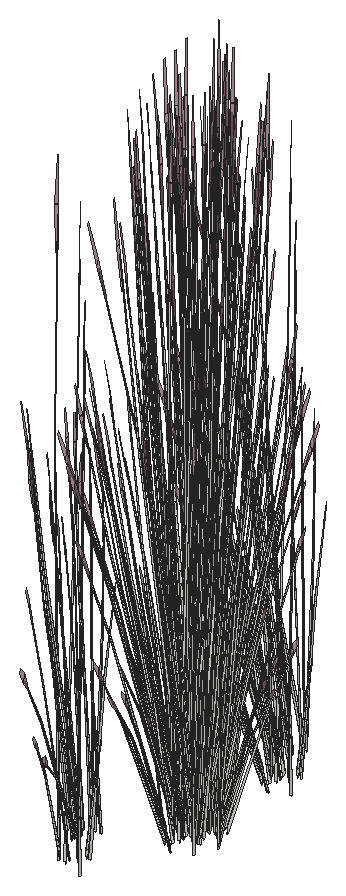
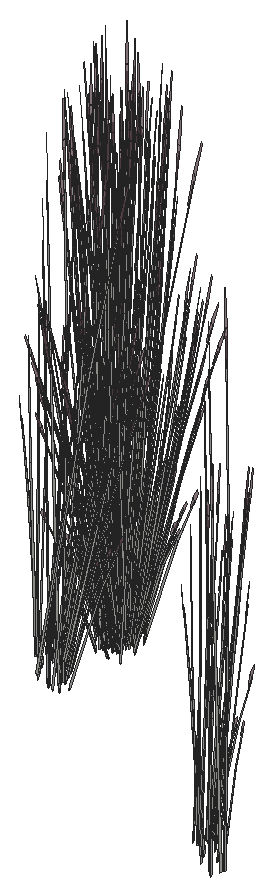
# SketchUp Ruby script. Lengths in inches.
U = 1.inch
M = Sketchup.active_model
def pt(a) = Geom::Point3d.new(a.map { |v| v * U })
def face(e, loops, mat)
  f = e.add_face(loops[0].map { |a| pt(a) })
  loops[1..].each { |l| e.add_face(l.map { |a| pt(a) }).erase! }
  f.material = f.back_material = mat if mat
  f
end
# faces: each face lists its corners as indices into pts; further lists are holes
def faces(e, pts, list, mat = nil) = list.each { |f| face(e, (f[0].is_a?(Array) ? f : [f]).map { |l| l.map { |i| pts[i] } }, mat) }
# xy, xz, yz: faces in a plane at the given z, y or x. An outline is a flat list of corners, or four numbers for a rectangle; further outlines are holes
def ring(l) = l.size == 4 ? [[l[0], l[1]], [l[2], l[1]], [l[2], l[3]], [l[0], l[3]]] : l.each_slice(2).to_a
def flat(e, list, mat, &to3) = list.each { |f| face(e, (f[0].is_a?(Array) ? f : [f]).map { |l| ring(l).map { |u, v| to3.(u, v) } }, mat) }
def xy(e, z, list, mat = nil) = flat(e, list, mat) { |x, y| [x, y, z] }
def xz(e, y, list, mat = nil) = flat(e, list, mat) { |x, z| [x, y, z] }
def yz(e, x, list, mat = nil) = flat(e, list, mat) { |y, z| [x, y, z] }
def lines(e, pts, list) = list.each { |a, b| e.add_line(pt(pts[a]), pt(pts[b])) }
# prism: a flat outline (further loops are holes) pulled along v
def prism(e, loops, v, mat = nil)
  f = face(e, loops, mat); d = Geom::Vector3d.new(v.map { |x| x * U })
  f.pushpull(f.normal.samedirection?(d) ? d.length : -d.length)
end
def box(e, o, s, mat = nil) = prism(e, [[o, [o[0] + s[0], o[1], o[2]], [o[0] + s[0], o[1] + s[1], o[2]], [o[0], o[1] + s[1], o[2]]]], [0, 0, s[2]], mat)
def at(x, y, z, deg = 0) = Geom::Transformation.translation(pt([x, y, z])) * Geom::Transformation.rotation(ORIGIN, Z_AXIS, deg.degrees)
def axes(o, x, y, z) = Geom::Transformation.new([*x, 0, *y, 0, *z, 0, *pt(o).to_a, 1])
def part(name) = M.definitions.add(name)
# library, detail: a bought-in or finely detailed component or shape, given as its bounding box
def library(name, o, s) = part(name).tap { |d| box(d.entities, o, s) }
def detail(e, o, s) = box(e.add_group.entities, o, s)
def put(e, d, t, mat = nil) = e.add_instance(d, t).tap { |i| i.material = mat if mat }
def group(e, t, mat = nil) = e.add_group.tap { |g| g.transformation = t; g.material = mat if mat }.entities
root = M.entities
M.materials.add("LightPink_Translucent").color = [144, 107, 117]
M.materials["LightPink_Translucent"].alpha = 0.75
c1 = part("blade")
p = [[2.15,0.21,22],[0,0.17,0],[0.09,0.45,0],[2.18,0.31,22],[2.29,0.31,22],[0.38,0.45,0],
  [2.48,0.24,33],[2.49,0.24,33],[2.48,0.22,33]]
faces(c1.entities,p,[[0,1,2,3],[4,5,2,3],[6,3,4,7],[8,0,3,6]])
c2 = part("seeds")
p = [[0.3,-0.1,1.38],[-0.01,-0.03,1.59],[-0.01,-0.03,0.03],[0.14,-0.07,-0.07],[0.29,-0.03,3],[0.15,0.01,3.11]]
faces(c2.entities,p,[[0,1,2,3],[1,0,4,5]],"LightPink_Translucent")
c3 = part("blade with seeds")
put(c3.entities,c1,at(0,0,0))
put(c3.entities,c2,axes([2.4,0.25,30.99],[1.5799,-0.05474,1.17369],[-0.12525,1.92788,0.29478],[-0.07173,-0.02425,1.56792]))
put(root,c3,axes([401.27,9.57,3.875],[0.08068,0.14973,1.71376],[-0.3728,0.12606,0.13857],[-0.08426,-0.23506,0.73262]))
put(root,c3,axes([402.72,9.36,2.59],[-0.10032,0.0944,1.43002],[-0.30046,-0.16522,-0.30754],[0.05569,-0.20547,0.61141]))
put(root,c3,axes([402.27,9.68,4.98],[-0.16845,-0.3792,-0.71045],[0.34676,-0.21133,0.08574],[-0.03939,-0.18322,1.00501]))
put(root,c3,axes([401.17,9.18,2.59],[-0.02137,0.15256,1.43002],[-0.31245,0.12771,-0.30754],[-0.07303,-0.19719,0.61141]))
put(root,c3,axes([401.98,8.84,1.49],[-0.0592,0.0168,1.76342],[-0.32738,-0.18913,-0.26939],[0.00549,-0.15776,0.30037]))
put(root,c3,axes([402.97,10.06,4.98],[0.00918,-0.43138,-0.71045],[0.38672,0.02897,0.08574],[0.04081,-0.18275,1.00501]))
put(root,c3,axes([402.3,9.36,4.53],[0.1064,-0.35863,-0.35414],[0.31043,0.1046,0.4572],[-0.02846,-0.14439,0.87481]))
put(root,c3,axes([402.53,9.84,3.875],[-0.06572,0.16029,1.71376],[-0.27569,-0.33172,0.13857],[0.12437,-0.20675,0.73262]))
put(root,c3,axes([402.14,9.61,4.68],[-0.34695,-0.11691,-0.51099],[0.11892,-0.40083,-0.3958],[-0.03181,-0.16138,0.97773]))
put(root,c3,axes([402.35,8.6,2.77],[0.04528,0.27194,1.1486],[-0.25117,-0.15062,0.84392],[0.02703,-0.13924,0.25299]))
put(root,c3,axes([402.89,9.91,4.68],[-0.25266,-0.31335,-0.51099],[0.2669,-0.27442,-0.3958],[0.03844,-0.15921,0.97773]))
put(root,c3,axes([403.13,9.8,4.53],[0.23881,-0.24554,-0.35414],[0.22606,0.28036,0.4572],[0.0344,-0.14245,0.87481]))
put(root,c3,axes([401.0625,8.93,2.77],[0.18411,0.16231,1.1486],[-0.26813,0.09757,0.84392],[-0.05737,-0.12474,0.25299]))
put(root,c3,axes([401.51,9.79,4.98],[-0.30095,-0.22541,-0.71045],[0.21388,-0.395,0.08574],[-0.10904,-0.13459,1.00501]))
put(root,c3,axes([401.4,9.49,4.53],[-0.05451,-0.37564,-0.35414],[0.31161,-0.09919,0.4572],[-0.0837,-0.10765,0.87481]))
put(root,c3,axes([400.92,9.42,1.49],[-0.03419,0.06144,1.76342],[-0.3455,0.13246,-0.26939],[-0.08346,-0.12049,0.30037]))
put(root,c3,axes([401.49,11.11,2.1],[-0.14494,-0.47823,-0.69835],[0.41752,-0.17223,-0.18329],[-0.01602,-0.16194,1.54149]))
put(root,c3,axes([400.73,10.04,3.875],[0.1311,0.08035,1.71376],[-0.27131,0.33708,0.13857],[-0.16909,-0.15206,0.73262]))
put(root,c3,axes([403.43,9.65,1.49],[-0.05283,-0.03674,1.76342],[-0.13569,-0.41045,-0.26939],[0.09154,-0.11138,0.30037]))
put(root,c3,axes([401.37,9.8,4.68],[-0.34827,0.11086,-0.51099],[-0.06092,-0.41983,-0.3958],[-0.09354,-0.12031,0.97773]))
put(root,c3,axes([403.42,10.81,4.98],[0.18436,-0.36797,-0.71045],[0.32306,0.26151,0.08574],[0.11008,-0.13332,1.00501]))
put(root,c3,axes([401.43,9.73,2.375],[-0.22066,-0.46731,0],[0.36918,-0.26061,-0.51607],[0.08408,-0.05936,1.63711]))
put(root,c3,axes([403.41,10.63,4.68],[-0.09067,-0.42583,-0.51099],[0.34336,-0.07449,-0.3958],[0.0984,-0.11438,0.97773]))
put(root,c3,axes([401.92,9.17,2.13],[-0.2439,0.26754,-0.03893],[-0.22348,-0.29302,-0.17649],[-0.01573,-0.08303,0.58215]))
put(root,c3,axes([402.23,12.34,3.33],[0.305,0.18805,1.51261],[-0.29879,0.40513,0.59816],[-0.13384,-0.24012,1.26806]))
put(root,c3,axes([400.63,11.04,2.02],[0,-0.46636,-0.49651],[0.39487,0,0],[0,-0.10622,1.57504]))
put(root,c3,axes([401.73,9.66,2.02],[0.33032,-0.23318,-0.49651],[0.19744,0.41812,0],[0.07523,-0.05311,1.57504]))
put(root,c3,axes([403.69,10.47,2.59],[-0.12609,-0.01381,1.43002],[-0.12917,-0.37055,-0.30754],[0.1549,-0.10482,0.61141]))
put(root,c3,axes([402.12,10.62,2.06],[0.23773,-0.35053,-0.62353],[0.29532,0.31785,-0.16365],[0.09526,-0.08744,1.37633]))
put(root,c3,axes([403.84,9.79,2.77],[-0.11756,0.2374,1.1486],[-0.10105,-0.31895,0.84392],[0.09709,-0.07992,0.25299]))
put(root,c3,axes([403.67,10.68,4.53],[0.30722,-0.06665,-0.35414],[0.08112,0.381,0.4572],[0.08804,-0.10234,0.87481]))
put(root,c3,axes([401.71,11.23,2.21],[0.17124,-0.42022,-0.44739],[0.35581,0.20224,0.21531],[0,-0.09687,1.43643]))
put(root,c3,axes([400.68,10.15,4.53],[-0.20082,-0.29199,-0.35414],[0.2293,-0.2764,0.4572],[-0.1165,-0.04206,0.87481]))
put(root,c3,axes([401.86,11.02,2.67],[-0.04113,-0.53214,-0.29095],[0.42835,-0.03218,-0.50002],[0.07543,-0.07088,1.59708]))
put(root,c3,axes([400.8,11.05,2.03],[0.24637,-0.29097,-0.30978],[0.24637,0.29097,0.30978],[0,-0.09372,1.38974]))
put(root,c3,axes([400.7,9.66,2.13],[-0.10181,0.3808,-0.03893],[-0.31336,-0.11714,-0.17649],[-0.04758,-0.06228,0.58215]))
put(root,c3,axes([401.67,11.58,2.67],[-0.39748,-0.22252,-0.29095],[0.19139,-0.46966,-0.50002],[-0.01249,-0.11531,1.59708]))
put(root,c3,axes([400.53,11.4,2.375],[-0.44133,0,0],[0,-0.52122,-0.51607],[0,-0.11871,1.63711]))
put(root,c3,axes([400.61,10.46,2.59],[0.06891,0.12984,1.43002],[-0.15879,0.35293,-0.30754],[-0.16304,-0.08436,0.61141]))
put(root,c3,axes([401.81,9.85,2.03],[0.32928,0.11539,-0.30978],[-0.08291,0.40636,0.30978],[0.06638,-0.04686,1.38974]))
put(root,c3,axes([400.89,10.35,4.98],[-0.35281,-0.01123,-0.71045],[0.0237,-0.47284,0.08574],[-0.14947,-0.0499,1.00501]))
put(root,c3,axes([400.875,11.26,2.33],[-0.32829,0.39208,0.30756],[-0.32849,-0.38796,-0.36492],[-0.01146,-0.11134,1.64885]))
put(root,c3,axes([401.92,11.44,2.43],[0.39767,0.22603,0.24065],[-0.19139,0.46966,0.50002],[0,-0.10827,1.60543]))
put(root,c3,axes([401.77,12.08,2.4375],[0.09355,-0.55261,-0.23429],[0.44354,0.09633,0.51271],[-0.0775,-0.07631,1.5644]))
put(root,c3,axes([400.78,10.45,4.68],[-0.25628,0.30892,-0.51099],[-0.22444,-0.32634,-0.3958],[-0.13021,-0.047,0.97773]))
put(root,c3,axes([400.2,10.85,2.77],[0.22533,-0.03337,1.1486],[-0.14293,0.29403,0.84392],[-0.11135,-0.04411,0.25299]))
put(root,c3,axes([401.79,11.125,2.72],[-0.38326,0.02879,0.44739],[-0.03466,-0.47788,-0.21531],[0.06861,-0.04843,1.43643]))
put(root,c3,axes([400.8,11.48,2.48],[0,0.46636,0.49651],[-0.39487,0,0],[0,-0.10622,1.57504]))
put(root,c3,axes([403.57,11.58,4.68],[0.09562,-0.42421,-0.51099],[0.32782,0.1454,-0.3958],[0.13199,-0.0389,0.97773]))
put(root,c3,axes([403.06,9.85,2.375],[0.22066,-0.46731,0],[0.36918,0.26061,-0.51607],[0.08408,0.05936,1.63711]))
put(root,c3,axes([400.46,10.78,3.875],[0.14639,-0.01056,1.71376],[-0.09712,0.45778,0.13857],[-0.20862,-0.02831,0.73262]))
put(root,c3,axes([401.73,11.85,2.21],[-0.21202,-0.39143,-0.44739],[0.32115,-0.27564,0.21531],[-0.06861,-0.04843,1.43643]))
put(root,c3,axes([401.78,11.3,2.36],[0.15345,0.52148,0.45755],[-0.43845,0.18134,0.17955],[0.00536,-0.09582,1.58856]))
put(root,c3,axes([403.92,11.7,1.98],[-0.22732,0.05597,1.41583],[-0.03618,-0.44548,0.08104],[0.15921,-0.06743,0.80566]))
put(root,c3,axes([404.34,11.3,2.26],[-0.21881,-0.29821,-0.06488],[0.23965,-0.27324,-0.29416],[0.0679,-0.01924,0.97024]))
put(root,c3,axes([401.7,11.71,2.72],[-0.17124,0.42022,0.44739],[-0.35581,-0.20224,-0.21531],[0,-0.09687,1.43643]))
put(root,c3,axes([402.33,11.34,2.21],[0,-0.53961,0],[0.44133,0,0],[0,0,1.79456]))
put(root,c3,axes([402.87,10.1,2.48],[-0.33032,-0.23318,0.49651],[0.19744,-0.41812,0],[0.07523,0.05311,1.57504]))
put(root,c3,axes([403.51,11.73,4.98],[0.31014,-0.20596,-0.71045],[0.17284,0.42397,0.08574],[0.14985,-0.04816,1.00501]))
put(root,c3,axes([401.54,12,2.06],[-0.36714,-0.07646,-0.62353],[0.07747,-0.47163,-0.16365],[-0.10956,-0.05715,1.37633]))
put(root,c3,axes([402.12,11,2.36],[-0.29264,0.42323,0.45755],[-0.34767,-0.3736,0.17955],[0.07055,-0.04224,1.58856]))
put(root,c3,axes([402.44,11.76,2.3],[-0.32829,-0.4014,-0.06131],[0.32849,-0.40164,0],[-0.01146,-0.01402,1.75571]))
put(root,c3,axes([401.61,10.31,2.47],[-0.10196,0.46348,0.17642],[-0.3731,-0.13116,0.35086],[0.06445,-0.00226,1.60407]))
put(root,c3,axes([401.46,10.68,1.59],[-0.3474,0.18671,1.28929],[-0.11057,-0.53572,0.50096],[0.21332,0.00891,1.46642]))
put(root,c3,axes([402.39,10.82,2.62],[0.06809,-0.4162,0.1448],[0.33266,0.07225,-0.41347],[0.06054,0.04274,1.26744]))
put(root,c3,axes([401.82,11.81,2.36],[0.44609,0.09826,0.45755],[-0.09078,0.55493,0.17955],[-0.06519,-0.05359,1.58856]))
put(root,c3,axes([404.17,11.41,1.49],[-0.01845,-0.0708,1.76342],[0.12793,-0.41416,-0.26939],[0.12905,-0.00596,0.30037]))
put(root,c3,axes([400.36,11.34,1.49],[0.00895,0.0735,1.76342],[-0.18044,0.38382,-0.26939],[-0.12817,-0.01935,0.30037]))
put(root,c3,axes([402.25,10.93,2.72],[-0.21202,-0.39143,0.44739],[0.32115,-0.27564,-0.21531],[0.06861,0.04843,1.43643]))
put(root,c3,axes([401.15,12.72,2.03],[-0.08291,-0.40636,-0.30978],[0.32928,-0.11539,0.30978],[-0.06638,-0.04686,1.38974]))
put(root,c3,axes([401.58,12.7,2.47],[0.37926,-0.12378,0.17642],[0.09365,0.46065,0.35086],[-0.03382,-0.06712,1.60407]))
put(root,c3,axes([402.36,10.96,2.67],[0.35635,-0.30962,-0.29095],[0.23697,0.43749,-0.50002],[0.08792,0.04443,1.59708]))
put(root,c3,axes([403.78,11.77,4.53],[0.29332,0.1301,-0.35414],[-0.08555,0.37955,0.4572],[0.11809,-0.0348,0.87481]))
put(root,c3,axes([401.0625,12.89,2.02],[-0.33032,-0.23318,-0.49651],[0.19744,-0.41812,0],[-0.07523,-0.05311,1.57504]))
put(root,c3,axes([403.26,10.13,2.02],[0.33032,0.23318,-0.49651],[-0.19744,0.41812,0],[0.07523,0.05311,1.57504]))
put(root,c3,axes([400.33,11.17,4.53],[-0.29332,-0.1301,-0.35414],[0.08555,-0.37955,0.4572],[-0.11809,0.0348,0.87481]))
put(root,c3,axes([402.63,11.46,2.21],[0.39487,0,0],[0,0.48281,0],[0,0,1.78407]))
put(root,c3,axes([401.96,12.07,2.67],[-0.35635,0.30962,-0.29095],[-0.23697,-0.43749,-0.50002],[-0.08792,-0.04443,1.59708]))
put(root,c3,axes([402.74,10.33,2.47],[-0.37926,0.12378,0.17642],[-0.09365,-0.46065,0.35086],[0.03382,0.06712,1.60407]))
put(root,c3,axes([402.98,11.3,3.875],[-0.14639,0.01056,1.71376],[0.09712,-0.45778,0.13857],[0.20862,0.02831,0.73262]))
put(root,c3,axes([403.17,10.31,2.03],[0.08291,0.40636,-0.30978],[-0.32928,0.11539,0.30978],[0.06638,0.04686,1.38974]))
put(root,c3,axes([402.5,11.22,2.38],[-0.44609,-0.09826,0.49198],[0.09078,-0.55493,0.19306],[0.06519,0.05359,1.70813]))
put(root,c3,axes([402.15,12.59,2.2],[-0.11516,-0.40207,0],[0.32884,-0.1408,0],[0,0,1.54371]))
put(root,c3,axes([401.93,12.21,2.62],[-0.06809,0.4162,0.1448],[-0.33266,-0.07225,-0.41347],[-0.06054,-0.04274,1.26744]))
put(root,c3,axes([402.58,12.53,2.18],[0.37054,-0.15823,-0.19198],[0.1302,0.45581,0.00008],[0.0409,-0.01749,1.73897]))
put(root,c3,axes([402.71,12.72,2.47],[0.10196,-0.46348,0.17642],[0.3731,0.13116,0.35086],[-0.06445,0.00226,1.60407]))
put(root,c3,axes([402.62,11.67,2.21],[0.24637,0.30123,0],[-0.24637,0.30123,0],[0,0,1.69266]))
put(root,c3,axes([401.22,11.1,3.34],[0.10032,-0.06746,1.77064],[0.0346,0.47103,0.13857],[-0.2173,0.0625,0.63284]))
put(root,c3,axes([403.29,11.54,2.47],[-0.2773,-0.3397,0.17642],[0.27945,-0.32949,0.35086],[-0.03063,0.06937,1.60407]))
put(root,c3,axes([402.78,11.03,2.06],[0.36714,0.07646,-0.62353],[-0.07747,0.47163,-0.16365],[0.10956,0.05715,1.37633]))
put(root,c3,axes([404.4,11.85,2.77],[-0.21807,0.07699,1.1486],[0.10265,-0.31819,0.84392],[0.11568,0.02177,0.25299]))
put(root,c3,axes([402.07,12.77,2.2],[-0.35581,-0.20937,0],[0.17124,-0.43505,0],[0,0,1.62707]))
put(root,c3,axes([402.36,12.21,2.46],[-0.34464,-0.37536,-0.25192],[0.29,-0.42149,0.5513],[-0.0928,0.04391,1.68216]))
put(root,c3,axes([401.45,12.93,2.48],[0.33032,0.23318,0.49651],[-0.19744,0.41812,0],[-0.07523,-0.05311,1.57504]))
put(root,c3,axes([402.62,11.32,2.72],[0.17124,-0.42022,0.44739],[0.35581,0.20224,-0.21531],[0,0.09687,1.43643]))
put(root,c3,axes([402.55,11.56,2.29],[0,0.53934,-0.05637],[-0.44133,0,0],[0,0.01695,1.79368]))
put(root,c3,axes([400.53,11.36,4.68],[-0.09562,0.42421,-0.51099],[-0.32782,-0.1454,-0.3958],[-0.13199,0.0389,0.97773]))
put(root,c3,axes([402.58,11.18,2.21],[0.21202,0.39143,-0.44739],[-0.32115,0.27564,0.21531],[0.06861,0.04843,1.43643]))
put(root,c3,axes([404.02,12.83,3.93],[-0.06755,-0.39203,-0.03492],[0.31928,-0.09013,-0.15832],[0.06667,0.02485,0.52218]))
put(root,c3,axes([401.26,13.18,2.375],[-0.22066,0.46731,0],[-0.36918,-0.26061,-0.51607],[-0.08408,-0.05936,1.63711]))
put(root,c3,axes([403.52,11.55,2.48],[0,-0.46636,0.49651],[0.39487,0,0],[0,0.10622,1.57504]))
put(root,c3,axes([402.53,11.9,2.72],[0.38326,-0.02879,0.44739],[0.03466,0.47788,-0.21531],[-0.06861,0.04843,1.43643]))
put(root,c3,axes([402.77,11.41,2.62],[0.32884,-0.136,0.1448],[0.11516,0.38837,-0.41347],[0,0.08547,1.26744]))
put(root,c3,axes([402.1875,12.13,2.21],[-0.38326,0.02879,-0.44739],[-0.03466,-0.47788,0.21531],[-0.06861,0.04843,1.43643]))
put(root,c3,axes([403.99,12.36,2.59],[-0.085,-0.1147,1.43002],[0.1106,-0.37943,-0.30754],[0.17198,0.0514,0.61141]))
put(root,c3,axes([402.47,12.78,2.2],[0.35581,0.20937,0],[-0.17124,0.43505,0],[0,0,1.74954]))
put(root,c3,axes([402.61,13.24,2.19],[-0.21791,-0.46895,-0.05142],[0.36918,-0.26061,0.51607],[-0.09097,0.04465,1.6363]))
put(root,c3,axes([402.53,12.11,2.62],[0.26075,0.2802,0.1448],[-0.2175,0.31612,-0.41347],[-0.06054,0.04274,1.26744]))
put(root,c3,axes([400.52,11.58,3.875],[0.12246,-0.09864,1.71376],[0.1031,0.45582,0.13857],[-0.19225,0.10302,0.73262]))
put(root,c3,axes([403.21,12.59,4.98],[0.35281,0.01123,-0.71045],[-0.0237,0.47284,0.08574],[0.14947,0.0499,1.00501]))
put(root,c3,axes([402.8125,12.97,2.48],[0.33032,-0.23318,0.49651],[0.19744,0.41812,0],[-0.07523,0.05311,1.57504]))
put(root,c3,axes([402.34,12.6,2.29],[0.15345,0.53576,-0.06012],[-0.43845,0.18773,0],[0.00536,0.01871,1.72173]))
put(root,c3,axes([402.51,13.18,2.03],[-0.32928,-0.11539,-0.30978],[0.08291,-0.40636,0.30978],[-0.06638,0.04686,1.38974]))
put(root,c3,axes([400.14,12.36,2.59],[0.12266,0.03828,1.43002],[0.07906,0.39104,-0.30754],[-0.16661,0.0732,0.61141]))
put(root,c3,axes([403.78,11.63,2.375],[0.44133,0,0],[0,0.52122,-0.51607],[0,0.11871,1.63711]))
put(root,c3,axes([403.61,11.9,2.2],[-0.44111,-0.00373,-0.04976],[0,-0.52122,0.49943],[-0.01386,0.11865,1.58352]))
put(root,c3,axes([402.65,11.45,2.67],[0.39748,0.22252,-0.29095],[-0.19139,0.46966,-0.50002],[0.01249,0.11531,1.59708]))
put(root,c3,axes([399.88,13.18,2.77],[0.14709,-0.21136,1.1486],[0.05804,0.3346,0.84392],[-0.1063,0.05991,0.25299]))
put(root,c3,axes([403.42,12.79,4.53],[0.20082,0.29199,-0.35414],[-0.2293,0.2764,0.4572],[0.1165,0.04206,0.87481]))
put(root,c3,axes([403.52,11.98,2.03],[-0.24637,0.29097,-0.30978],[-0.24637,-0.29097,0.30978],[0,0.09372,1.38974]))
put(root,c3,axes([402.46,12,2.67],[0.04113,0.53214,-0.29095],[-0.42835,0.03218,-0.50002],[-0.07543,0.07088,1.59708]))
put(root,c3,axes([402.61,11.8,2.21],[-0.17124,0.42022,-0.44739],[-0.35581,-0.20224,0.21531],[0,0.09687,1.43643]))
put(root,c3,axes([400.43,12.26,4.53],[-0.30722,0.06665,-0.35414],[-0.08112,-0.381,0.4572],[-0.08804,0.10234,0.87481]))
put(root,c3,axes([402.2,12.41,2.06],[-0.23773,0.35053,-0.62353],[-0.29532,-0.31785,-0.16365],[-0.09526,0.08744,1.37633]))
put(root,c3,axes([402.62,13,2.33],[0.44186,0.15158,0.30756],[-0.11054,0.54181,-0.36492],[-0.07313,0.06781,1.64885]))
put(root,c3,axes([402.59,13.37,2.02],[-0.33032,0.23318,-0.49651],[-0.19744,-0.41812,0],[-0.07523,0.05311,1.57504]))
put(root,c3,axes([403.6875,11.99,2.02],[0,0.46636,-0.49651],[-0.39487,0,0],[0,0.10622,1.57504]))
put(root,c3,axes([402.7,12.04,3.875],[-0.1311,-0.08035,1.71376],[0.27131,-0.33708,0.13857],[0.16909,0.15206,0.73262]))
put(root,c3,axes([403.18,12.95,2.77],[-0.19872,-0.13409,1.1486],[0.2566,-0.13625,0.84392],[0.06921,0.11541,0.25299]))
put(root,c3,axes([400.97,11.89,3.875],[0.08815,-0.14329,1.71376],[0.22258,0.38678,0.13857],[-0.15267,0.17614,0.73262]))
put(root,c3,axes([400.6875,12.31,4.68],[0.09067,0.42583,-0.51099],[-0.34336,0.07449,-0.3958],[-0.0984,0.11438,0.97773]))
put(root,c3,axes([402.89,13.29,2.375],[0.22066,0.46731,0],[-0.36918,0.26061,-0.51607],[-0.08408,0.05936,1.63711]))
put(root,c3,axes([403.24,13.45,1.49],[0.02571,-0.06733,1.76342],[0.32373,-0.19829,-0.26939],[0.09815,0.10263,0.30037]))
put(root,c3,axes([402.7,11.44,2.84],[-0.00964,-0.43909,1.41272],[0.43635,0.11382,0.59816],[-0.1032,0.24027,1.3335]))
put(root,c3,axes([402.8125,11.92,2.09],[0.12941,0.42699,-0.69212],[-0.37279,0.15378,-0.18165],[0.0143,0.14459,1.52773]))
put(root,c3,axes([400.27,13.39,1.49],[0.04734,0.04659,1.76342],[0.08027,0.4317,-0.26939],[-0.10492,0.09206,0.30037]))
put(root,c3,axes([402.74,13.14,4.68],[0.34827,-0.11086,-0.51099],[0.06092,0.41983,-0.3958],[0.09354,0.12031,0.97773]))
put(root,c3,axes([403.22,13.5625,2.67],[-0.22633,-0.01463,1.0506],[0.14947,-0.31064,0.58006],[0.08941,0.11036,0.8241]))
put(root,c3,axes([400.9,12.24,3.875],[0.06572,-0.16029,1.71376],[0.27569,0.33172,0.13857],[-0.12437,0.20675,0.73262]))
put(root,c3,axes([402.48,12.81,2.59],[0.00623,-0.15459,1.43002],[0.29764,-0.17268,-0.30754],[0.09188,0.18503,0.61141]))
put(root,c3,axes([400.98,13.14,4.53],[-0.23881,0.24554,-0.35414],[-0.22606,-0.28036,0.4572],[-0.0344,0.14245,0.87481]))
put(root,c3,axes([401.13,14.1,2.77],[-0.00913,-0.2773,1.1486],[0.22824,0.19778,0.84392],[-0.04489,0.13217,0.25299]))
put(root,c3,axes([401.73,13.4375,1.49],[0.05712,-0.02538,1.76342],[0.34359,0.13968,-0.26939],[0.01005,0.15742,0.30037]))
put(root,c3,axes([401.21,13.03,5],[0.25266,0.31335,-0.5672],[-0.2669,0.27442,-0.43934],[-0.03844,0.15921,1.08528]))
put(root,c3,axes([400.9375,13.5,2.82],[0.32063,-0.08258,0.06507],[0.07371,0.33271,-0.86304],[-0.02033,0.16842,0.7736]))
put(root,c3,axes([401.27,20.52,3.875],[0.08068,0.14973,1.71376],[-0.3728,0.12606,0.13857],[-0.08426,-0.23506,0.73262]))
put(root,c3,axes([401.96,13.33,4.68],[0.34695,0.11691,-0.51099],[-0.11892,0.40083,-0.3958],[0.03181,0.16138,0.97773]))
put(root,c3,axes([402.16,12.5,3.875],[-0.08068,-0.14973,1.71376],[0.3728,-0.12606,0.13857],[0.08426,0.23506,0.73262]))
put(root,c3,axes([383.7,20.3,-10.62],[-0.10032,0.0944,1.43002],[-0.30046,-0.16522,-0.30754],[0.05569,-0.20547,0.61141]))
put(root,c3,axes([402.72,20.3,2.59],[-0.10032,0.0944,1.43002],[-0.30046,-0.16522,-0.30754],[0.05569,-0.20547,0.61141]))
put(root,c3,axes([401.8,13.58,4.53],[-0.1064,0.35863,-0.35414],[-0.31043,-0.1046,0.4572],[0.02846,0.14439,0.87481]))
put(root,c3,axes([402.27,20.63,4.98],[-0.16845,-0.3792,-0.71045],[0.34676,-0.21133,0.08574],[-0.03939,-0.18322,1.00501]))
put(root,c3,axes([401.17,20.12,2.59],[-0.02137,0.15256,1.43002],[-0.31245,0.12771,-0.30754],[-0.07303,-0.19719,0.61141]))
put(root,c3,axes([401.13,12.89,5.34],[-0.00918,0.43138,-0.7886],[-0.38672,-0.02897,0.09517],[-0.04081,0.18275,1.11556]))
put(root,c3,axes([401.98,19.79,1.49],[-0.0592,0.0168,1.76342],[-0.32738,-0.18913,-0.26939],[0.00549,-0.15776,0.30037]))
put(root,c3,axes([401.5,12.58,3.875],[-0.00864,-0.17899,1.71376],[0.37441,0.11874,0.13857],[-0.02316,0.25508,0.73262]))
put(root,c3,axes([383.9375,21,-8.23],[0.00918,-0.43138,-0.71045],[0.38672,0.02897,0.08574],[0.04081,-0.18275,1.00501]))
put(root,c3,axes([402.97,21,4.98],[0.00918,-0.43138,-0.71045],[0.38672,0.02897,0.08574],[0.04081,-0.18275,1.00501]))
put(root,c3,axes([401.84,13.26,4.98],[0.16845,0.3792,-0.71045],[-0.34676,0.21133,0.08574],[0.03939,0.18322,1.00501]))
put(root,c3,axes([384.48,20.33,-8.5],[-0.00341,-0.09282,1.74944],[-0.28775,-0.26825,-0.27667],[0.04449,-0.16261,0.14031]))
put(root,c3,axes([402.3,20.31,4.53],[0.1064,-0.35863,-0.35414],[0.31043,0.1046,0.4572],[-0.02846,-0.14439,0.87481]))
put(root,c3,axes([383.5,20.78,-9.33],[-0.06572,0.16029,1.71376],[-0.27569,-0.33172,0.13857],[0.12437,-0.20675,0.73262]))
put(root,c3,axes([402.53,20.78,3.875],[-0.06572,0.16029,1.71376],[-0.27569,-0.33172,0.13857],[0.12437,-0.20675,0.73262]))
put(root,c3,axes([384.4,19.99,-8.5],[-0.03584,0.03562,1.77383],[-0.35118,-0.12018,-0.16761],[-0.01271,-0.15545,0.31391]))
put(root,c3,axes([400.86,13.85,2.59],[0.11138,-0.07357,1.43002],[0.27499,0.22183,-0.30754],[-0.08185,0.19194,0.61141]))
put(root,c3,axes([402.14,20.55,4.68],[-0.34695,-0.11691,-0.51099],[0.11892,-0.40083,-0.3958],[-0.03181,-0.16138,0.97773]))
put(root,c3,axes([383.33,19.55,-10.45],[0.04528,0.27194,1.1486],[-0.25117,-0.15062,0.84392],[0.02703,-0.13924,0.25299]))
put(root,c3,axes([402.35,19.55,2.77],[0.04528,0.27194,1.1486],[-0.25117,-0.15062,0.84392],[0.02703,-0.13924,0.25299]))
put(root,c3,axes([383.86,20.86,-8.53],[-0.25266,-0.31335,-0.51099],[0.2669,-0.27442,-0.3958],[0.03844,-0.15921,0.97773]))
put(root,c3,axes([402.89,20.86,4.68],[-0.25266,-0.31335,-0.51099],[0.2669,-0.27442,-0.3958],[0.03844,-0.15921,0.97773]))
put(root,c3,axes([383.31,20.39,-8.48],[0.34777,0.12192,0.48003],[-0.11892,0.40083,0.3958],[-0.0209,-0.15763,0.9933]))
put(root,c3,axes([401.01,13.49,3.36],[0.00775,-0.24075,1.54345],[0.34877,0.12716,0.21329],[-0.03022,0.25658,0.72882]))
put(root,c3,axes([384.125,21.02,-8.18],[-0.3879,-0.02311,-0.1216],[0.0106,-0.43749,-0.67495],[0.02694,-0.1685,1.02557]))
put(root,c3,axes([384.1,20.74,-8.68],[0.23881,-0.24554,-0.35414],[0.22606,0.28036,0.4572],[0.0344,-0.14245,0.87481]))
put(root,c3,axes([403.13,20.74,4.53],[0.23881,-0.24554,-0.35414],[0.22606,0.28036,0.4572],[0.0344,-0.14245,0.87481]))
put(root,c3,axes([401.0625,19.875,2.77],[0.18411,0.16231,1.1486],[-0.26813,0.09757,0.84392],[-0.05737,-0.12474,0.25299]))
put(root,c3,axes([401.51,20.74,4.98],[-0.30095,-0.22541,-0.71045],[0.21388,-0.395,0.08574],[-0.10904,-0.13459,1.00501]))
put(root,c3,axes([401.4,20.4375,4.53],[-0.05451,-0.37564,-0.35414],[0.31161,-0.09919,0.4572],[-0.0837,-0.10765,0.87481]))
put(root,c3,axes([400.92,20.37,1.49],[-0.03419,0.06144,1.76342],[-0.3455,0.13246,-0.26939],[-0.08346,-0.12049,0.30037]))
put(root,c3,axes([401.49,22.05,2.1],[-0.14494,-0.47823,-0.69835],[0.41752,-0.17223,-0.18329],[-0.01602,-0.16194,1.54149]))
put(root,c3,axes([400.73,20.98,3.875],[0.1311,0.08035,1.71376],[-0.27131,0.33708,0.13857],[-0.16909,-0.15206,0.73262]))
put(root,c3,axes([384.4,20.59,-11.72],[-0.05283,-0.03674,1.76342],[-0.13569,-0.41045,-0.26939],[0.09154,-0.11138,0.30037]))
put(root,c3,axes([403.43,20.59,1.49],[-0.05283,-0.03674,1.76342],[-0.13569,-0.41045,-0.26939],[0.09154,-0.11138,0.30037]))
put(root,c3,axes([401.37,20.75,4.68],[-0.34827,0.11086,-0.51099],[-0.06092,-0.41983,-0.3958],[-0.09354,-0.12031,0.97773]))
put(root,c3,axes([384.1,20.84,-8.48],[0.25132,0.3182,0.48003],[-0.2669,0.27442,0.3958],[0.04636,-0.14929,0.9933]))
put(root,c3,axes([384.19,20.87,-8.48],[0.29004,0.02173,0.0643],[-0.00795,0.32812,0.50621],[0.03035,-0.12569,0.77189]))
put(root,c3,axes([383.97,21.09,-8.16],[-0.23881,0.24554,0.35414],[-0.22606,-0.28036,-0.4572],[0.0344,-0.14245,0.87481]))
put(root,c3,axes([384.39,21.75,-8.23],[0.18436,-0.36797,-0.71045],[0.32306,0.26151,0.08574],[0.11008,-0.13332,1.00501]))
put(root,c3,axes([403.42,21.75,4.98],[0.18436,-0.36797,-0.71045],[0.32306,0.26151,0.08574],[0.11008,-0.13332,1.00501]))
put(root,c3,axes([382.4,20.68,-10.84],[-0.22066,-0.46731,0],[0.36918,-0.26061,-0.51607],[0.08408,-0.05936,1.63711]))
put(root,c3,axes([401.43,20.68,2.375],[-0.22066,-0.46731,0],[0.36918,-0.26061,-0.51607],[0.08408,-0.05936,1.63711]))
put(root,c3,axes([384.39,21.58,-8.53],[-0.09067,-0.42583,-0.51099],[0.34336,-0.07449,-0.3958],[0.0984,-0.11438,0.97773]))
put(root,c3,axes([403.41,21.58,4.68],[-0.09067,-0.42583,-0.51099],[0.34336,-0.07449,-0.3958],[0.0984,-0.11438,0.97773]))
put(root,c3,axes([401.92,20.12,2.13],[-0.2439,0.26754,-0.03893],[-0.22348,-0.29302,-0.17649],[-0.01573,-0.08303,0.58215]))
put(root,c3,axes([384.55,21.88,-8.18],[-0.32648,-0.25715,-0.1216],[0.18809,-0.3724,-0.67495],[0.09224,-0.12945,1.02557]))
put(root,c3,axes([402.23,23.29,3.33],[0.305,0.18805,1.51261],[-0.29879,0.40513,0.59816],[-0.13384,-0.24012,1.26806]))
put(root,c3,axes([400.63,21.99,2.02],[0,-0.46636,-0.49651],[0.39487,0,0],[0,-0.10622,1.57504]))
put(root,c3,axes([382.7,20.61,-11.19],[0.33032,-0.23318,-0.49651],[0.19744,0.41812,0],[0.07523,-0.05311,1.57504]))
put(root,c3,axes([401.73,20.61,2.02],[0.33032,-0.23318,-0.49651],[0.19744,0.41812,0],[0.07523,-0.05311,1.57504]))
put(root,c3,axes([384.66,21.41,-10.62],[-0.12609,-0.01381,1.43002],[-0.12917,-0.37055,-0.30754],[0.1549,-0.10482,0.61141]))
put(root,c3,axes([403.69,21.41,2.59],[-0.12609,-0.01381,1.43002],[-0.12917,-0.37055,-0.30754],[0.1549,-0.10482,0.61141]))
put(root,c3,axes([385.35,21.77,-8.5],[-0.0461,-0.00354,1.77383],[-0.19143,-0.37951,-0.16761],[0.07688,-0.12478,0.31391]))
put(root,c3,axes([383.09,21.5625,-11.15],[0.23773,-0.35053,-0.62353],[0.29532,0.31785,-0.16365],[0.09526,-0.08744,1.37633]))
put(root,c3,axes([402.12,21.5625,2.06],[0.23773,-0.35053,-0.62353],[0.29532,0.31785,-0.16365],[0.09526,-0.08744,1.37633]))
put(root,c3,axes([384.81,20.73,-10.45],[-0.11756,0.2374,1.1486],[-0.10105,-0.31895,0.84392],[0.09709,-0.07992,0.25299]))
put(root,c3,axes([403.84,20.73,2.77],[-0.11756,0.2374,1.1486],[-0.10105,-0.31895,0.84392],[0.09709,-0.07992,0.25299]))
put(root,c3,axes([384.64,21.62,-8.68],[0.30722,-0.06665,-0.35414],[0.08112,0.381,0.4572],[0.08804,-0.10234,0.87481]))
put(root,c3,axes([403.67,21.62,4.53],[0.30722,-0.06665,-0.35414],[0.08112,0.381,0.4572],[0.08804,-0.10234,0.87481]))
put(root,c3,axes([401.71,22.18,2.21],[0.17124,-0.42022,-0.44739],[0.35581,0.20224,0.21531],[0,-0.09687,1.43643]))
